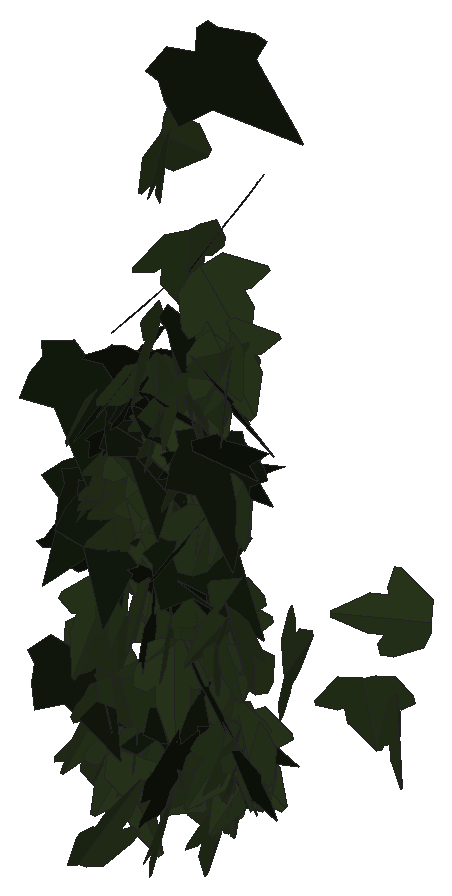
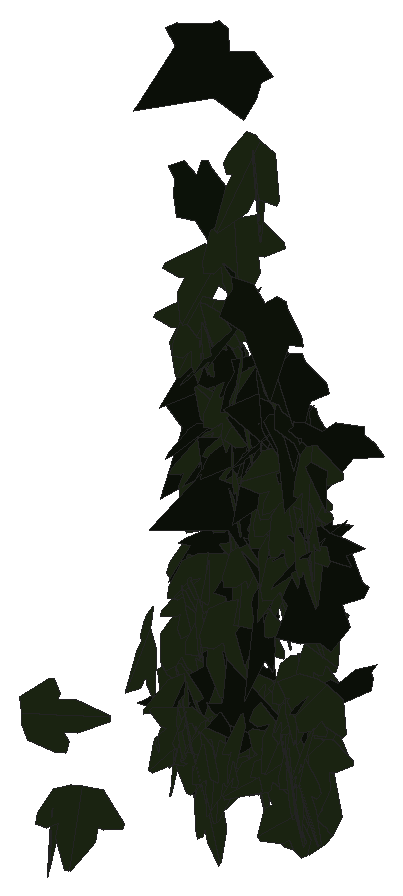
# SketchUp Ruby script. Lengths in inches.
U = 1.inch
M = Sketchup.active_model
def pt(a) = Geom::Point3d.new(a.map { |v| v * U })
def face(e, loops, mat)
  f = e.add_face(loops[0].map { |a| pt(a) })
  loops[1..].each { |l| e.add_face(l.map { |a| pt(a) }).erase! }
  f.material = f.back_material = mat if mat
  f
end
# faces: each face lists its corners as indices into pts; further lists are holes
def faces(e, pts, list, mat = nil) = list.each { |f| face(e, (f[0].is_a?(Array) ? f : [f]).map { |l| l.map { |i| pts[i] } }, mat) }
# xy, xz, yz: faces in a plane at the given z, y or x. An outline is a flat list of corners, or four numbers for a rectangle; further outlines are holes
def ring(l) = l.size == 4 ? [[l[0], l[1]], [l[2], l[1]], [l[2], l[3]], [l[0], l[3]]] : l.each_slice(2).to_a
def flat(e, list, mat, &to3) = list.each { |f| face(e, (f[0].is_a?(Array) ? f : [f]).map { |l| ring(l).map { |u, v| to3.(u, v) } }, mat) }
def xy(e, z, list, mat = nil) = flat(e, list, mat) { |x, y| [x, y, z] }
def xz(e, y, list, mat = nil) = flat(e, list, mat) { |x, z| [x, y, z] }
def yz(e, x, list, mat = nil) = flat(e, list, mat) { |y, z| [x, y, z] }
def lines(e, pts, list) = list.each { |a, b| e.add_line(pt(pts[a]), pt(pts[b])) }
# prism: a flat outline (further loops are holes) pulled along v
def prism(e, loops, v, mat = nil)
  f = face(e, loops, mat); d = Geom::Vector3d.new(v.map { |x| x * U })
  f.pushpull(f.normal.samedirection?(d) ? d.length : -d.length)
end
def box(e, o, s, mat = nil) = prism(e, [[o, [o[0] + s[0], o[1], o[2]], [o[0] + s[0], o[1] + s[1], o[2]], [o[0], o[1] + s[1], o[2]]]], [0, 0, s[2]], mat)
def at(x, y, z, deg = 0) = Geom::Transformation.translation(pt([x, y, z])) * Geom::Transformation.rotation(ORIGIN, Z_AXIS, deg.degrees)
def axes(o, x, y, z) = Geom::Transformation.new([*x, 0, *y, 0, *z, 0, *pt(o).to_a, 1])
def part(name) = M.definitions.add(name)
# library, detail: a bought-in or finely detailed component or shape, given as its bounding box
def library(name, o, s) = part(name).tap { |d| box(d.entities, o, s) }
def detail(e, o, s) = box(e.add_group.entities, o, s)
def put(e, d, t, mat = nil) = e.add_instance(d, t).tap { |i| i.material = mat if mat }
def group(e, t, mat = nil) = e.add_group.tap { |g| g.transformation = t; g.material = mat if mat }.entities
root = M.entities
M.materials.add("efeu1").color = [18, 25, 13]
M.materials.add("efeu2").color = [43, 57, 29]
c1 = part("ivyleaf_10")
p = [[0,0.5,-0.03],[-0.0625,2.02,-0.43],[-0.19,2.01,-0.46],[-0.54,1.05,-0.29],[-0.52,0.625,-0.18],[-0.83,0.76,-0.28],
  [-1.16,0.64,-0.33],[-1.15,0.33,-0.24],[-0.77,-0.39,0.02],[-0.3,-0.51,0.16],[0.04,-0.48,0.23],[-0.02,2.01,-0.4375],
  [-0.06,2.01,-0.43],[0.04,-0.49,0.23],[0.67,-0.49,0.14],[1.38,0.36,-0.2],[1.375,0.51,-0.24],[0.81,0.65,-0.19],
  [0.62,0.59,-0.15],[0.6,1.09,-0.28],[0.5,1.23,-0.31]]
faces(c1.entities,p,[[0,1,2,3,4,5,6,7,8,9,10],[11,12,0,13,14,15,16,17,18,19,20]],"efeu2")
c2 = part("ivyleaf_9")
p = [[1.54,2.16,1.25],[1.36,2.04,1.19],[-0.21,0.99,0.68],[-0.71,1.11,0.82],[-0.85,0.86,0.67],[-0.8,0.17,0.21],
  [-0.9,-0.01,0.1],[-0.67,-0.16,-0.02],[-0.08,-0.08,-0.05],[-0.03,-0.6,-0.4],[0.65,-0.88,-0.66],[0.83,-0.6,-0.49],
  [1.29,-0.42,-0.43],[1.8125,-0.07,-0.26],[1.21,0.44,0.15]]
faces(c2.entities,p,[[0,1,2,3,4,5,6,7,8,9,10,11,12,13,14]],"efeu1")
put(root,c1,axes([528.03,135.62,182.96],[0.04997,-0.69827,0.35422],[0.08449,0.35768,0.69317],[-0.77841,-0.006,0.09798]))
put(root,c1,axes([529.61,135.92,187.42],[0.72469,-0.04449,0.22869],[0.2279,-0.01976,-0.72603],[0.04837,0.75966,-0.0055]))
put(root,c1,axes([528.9,136.29,194.03],[0.25276,-0.34799,0.63465],[0.37642,-0.51097,-0.43009],[0.61821,0.4534,0.0024]))
put(root,c1,axes([529.51,135.85,184.14],[0.33931,-0.66324,-0.11644],[-0.04396,0.10828,-0.74493],[0.67195,0.342,0.01006]))
put(root,c1,axes([530.07,135.85,196.52],[-0.29708,-0.72355,-0.03236],[0.00307,0.03372,-0.7821],[0.72427,-0.29693,-0.00996]))
put(root,c2,axes([529.02,135.63,193.63],[-0.35835,0.68144,0.00431],[-0.00194,0.00385,-0.76992],[-0.68145,-0.35835,-0.00007]))
put(root,c2,axes([528.0625,136.24,189.86],[-0.09573,-0.76291,0.03566],[-0.00925,-0.03478,-0.76887],[0.76368,-0.09605,-0.00484]))
put(root,c1,axes([530.85,135.84,194.17],[-0.33415,-0.69594,-0.06383],[0.02014,0.06113,-0.77196],[0.69857,-0.33466,-0.00827]))
put(root,c1,axes([530.79,135.96,194.42],[0.72889,-0.26896,-0.11241],[-0.11049,0.02521,-0.77679],[0.26976,0.73707,-0.01445]))
put(root,c2,axes([530.46,135.66,187.6],[0.61618,-0.18002,-0.4099],[-0.39326,0.11558,-0.64194],[0.21393,0.73098,0.00055]))
put(root,c1,axes([528.93,135.89,188.72],[0.50162,-0.56592,-0.14151],[-0.06119,0.13455,-0.75503],[0.58012,0.50353,0.04271]))
put(root,c2,axes([529.75,135.23,184.89],[0.11701,0.22287,0.77167],[0.25966,0.72745,-0.24947],[-0.76008,0.28282,0.03357]))
put(root,c2,axes([528.97,136.23,192.11],[0.02537,-0.77043,-0.00224],[0.0001,0.00225,-0.77085],[0.77043,0.02537,0.00018]))
put(root,c1,axes([529.53,135.83,198.48],[0.37198,-0.66538,-0.21572],[-0.02506,0.23149,-0.75724],[0.69902,0.36238,0.08764]))
put(root,c2,axes([531.18,135.74,197.48],[-0.37583,0.69191,-0.09076],[0.04527,-0.0787,-0.78739],[-0.69637,-0.37854,-0.00221]))
put(root,c1,axes([529.17,135.92,193.36],[-0.39,-0.67294,-0.075],[0.08819,0.03533,-0.77559],[0.67133,-0.39557,0.05832]))
put(root,c1,axes([529.33,135.96,191.46],[-0.5995,-0.44929,0.13192],[-0.10238,-0.08335,-0.74915],[0.45692,-0.60816,0.00522]))
put(root,c1,axes([530.89,135.93,193.89],[0.52139,-0.58398,-0.08529],[0.04954,0.15671,-0.77016],[0.5881,0.50454,0.14049]))
put(root,c2,axes([530.53,135.64,200.75],[-0.06948,-0.12915,-0.8626],[0.43398,0.74549,-0.14658],[0.75658,-0.43948,0.00486]))
put(root,c1,axes([529.35,136.1,192.375],[0.26076,-0.72266,0.08953],[0.02445,-0.08636,-0.76825],[0.72778,0.26183,-0.00627]))
put(root,c1,axes([527.51,136.42,187.68],[-0.1066,-0.48141,0.55439],[0.28284,-0.54389,-0.41791],[0.67757,0.1513,0.26167]))
put(root,c2,axes([527.46,136.17,192.83],[-0.4125,-0.54509,-0.36487],[0.22909,0.28415,-0.68351],[0.61463,-0.47174,0.00989]))
put(root,c1,axes([529.62,135.74,193.27],[0.3847,-0.29258,-0.59439],[-0.40569,0.43936,-0.47883],[0.52376,0.55521,0.06569]))
put(root,c2,axes([530.5,136.21,192.05],[0.04603,-0.75714,-0.1445],[-0.01125,0.14409,-0.75853],[0.77073,0.04732,-0.00244]))
put(root,c1,axes([529.96,135.9,193.46],[-0.58466,0.51066,-0.08668],[0.06952,-0.05216,-0.77625],[-0.51327,-0.58874,-0.0064]))
put(root,c2,axes([527.22,136,186.73],[0.15379,-0.64621,-0.38759],[-0.0269,0.39062,-0.66193],[0.75305,0.14593,0.05551]))
put(root,c1,axes([527.78,136.29,185.7],[0.08487,0.5669,-0.472],[-0.26058,-0.42144,-0.55304],[-0.69012,0.22885,0.15077]))
put(root,c2,axes([530.27,135.87,193.9],[0.74862,-0.18729,-0.03452],[-0.03313,0.00981,-0.77169],[0.18754,0.74935,0.00147]))
put(root,c1,axes([530.96,136.07,191.26],[0.66168,-0.34231,-0.13025],[-0.10897,0.07277,-0.74484],[0.34966,0.67044,0.01435]))
put(root,c1,axes([528.38,135.85,188.53],[0.34681,-0.3359,-0.57591],[-0.42691,0.38674,-0.48265],[0.5121,0.54989,-0.01234]))
put(root,c1,axes([529.46,136.22,190.63],[-0.48763,-0.57572,0.15636],[0.0196,-0.2173,-0.73897],[0.59625,-0.46369,0.15216]))
put(root,c1,axes([529.02,136.1,191.6],[0.52098,0.5584,-0.11091],[-0.08551,-0.07188,-0.76358],[-0.56285,0.52779,0.01335]))
put(root,c2,axes([528.375,135.72,192.74],[-0.27222,0.69051,0.18515],[-0.08322,0.16617,-0.74206],[-0.71005,-0.2842,0.01599]))
put(root,c2,axes([527.84,136.42,190.25],[-0.67175,-0.3612,-0.01235],[0.01123,0.00519,-0.76271],[0.36124,-0.67185,0.00075]))
put(root,c1,axes([528.71,136.18,190.59],[-0.20937,-0.74045,0.0741],[-0.00139,-0.07659,-0.76923],[0.74414,-0.20847,0.01941]))
put(root,c1,axes([530.27,136.25,190.44],[-0.42889,-0.59636,0.21067],[-0.0606,-0.21463,-0.73091],[0.62957,-0.42692,0.07317]))
put(root,c2,axes([528.71,136.16,192.4],[0.25455,-0.68257,-0.23231],[0.01088,0.24997,-0.72254],[0.72094,0.23723,0.09293]))
put(root,c1,axes([528.48,136.29,189.77],[-0.11758,-0.7354,0.18371],[-0.00195,-0.18561,-0.74427],[0.758,-0.11455,0.02659]))
put(root,c1,axes([530.52,136.65,188.51],[0.05898,-0.24793,0.70378],[0.16298,-0.68465,-0.25484],[0.72815,0.17332,0.00004]))
put(root,c1,axes([530.69,136.4,185.81],[0.23583,0.47254,-0.49065],[-0.26364,-0.41545,-0.52682],[-0.62811,0.35179,0.03691]))
put(root,c2,axes([528.9,136.23,192.41],[0.51449,-0.57132,0.06293],[0.08496,-0.00793,-0.76667],[0.56846,0.51827,0.05764]))
put(root,c2,axes([529.85,136.1,194.64],[0.5184,-0.54014,-0.2023],[-0.09078,0.19221,-0.7458],[0.56959,0.52222,0.06526]))
put(root,c2,axes([530.13,135.85,190.32],[-0.29549,0.69132,0.10974],[-0.06843,0.09002,-0.75133],[-0.69662,-0.30208,0.02725]))
put(root,c2,axes([527.55,136.41,190.07],[0.14138,-0.74677,-0.04956],[0.02073,0.05432,-0.75943],[0.74813,0.13961,0.03041]))
put(root,c1,axes([529.43,136.16,191.8],[-0.57916,-0.4464,-0.25896],[0.33107,-0.02278,-0.70116],[0.39588,-0.63401,0.20752]))
put(root,c1,axes([529.73,136.125,192.91],[-0.36238,-0.6775,-0.10906],[0.04795,0.09803,-0.76832],[0.68455,-0.36552,-0.00392]))
put(root,c2,axes([528.93,135.93,193.67],[0.25115,0.63308,-0.36755],[-0.35506,-0.23447,-0.64646],[-0.64017,0.37841,0.21435]))
put(root,c1,axes([530.8,135.91,194.47],[0.36207,0.61508,0.32751],[0.08867,0.32541,-0.70917],[-0.69117,0.36396,0.08058]))
put(root,c2,axes([528.73,135.59,192.36],[-0.22363,0.72543,-0.3368],[-0.19552,0.28952,0.75342],[0.77553,0.28217,0.09283]))
put(root,c1,axes([529.78,135.91,191.94],[0.55958,0.2124,-0.49753],[0.43918,0.2396,0.59624],[0.31587,-0.70941,0.05241]))
put(root,c1,axes([530.59,135.9,195.76],[0.28328,0.64872,0.34617],[0.0998,0.33362,-0.70686],[-0.7285,0.29796,0.03777]))
put(root,c1,axes([528.43,136.24,190.9],[-0.27451,-0.70599,-0.01567],[0.01029,0.01282,-0.75747],[0.70609,-0.27465,0.00494]))
put(root,c1,axes([528.42,136.3,191.43],[-0.14221,-0.75335,0.02688],[-0.00755,-0.02593,-0.76665],[0.75379,-0.14238,-0.00261]))
put(root,c1,axes([529.17,136.19,192.53],[0.39766,-0.64727,-0.14511],[0.0143,0.17751,-0.75262],[0.66318,0.38429,0.10323]))
put(root,c2,axes([530.32,135.82,192.09],[0.62969,0.41873,0.08048],[0.08001,0.02495,-0.75584],[-0.41882,0.63432,-0.0234]))
put(root,c2,axes([529.03,135.92,192.73],[0.77179,0.05925,-0.00001],[-0.00778,0.10124,-0.76737],[-0.05874,0.76512,0.10154]))
put(root,c2,axes([529.51,135.97,188.96],[0.49836,0.36695,-0.44053],[-0.43808,-0.13283,-0.60623],[-0.36986,0.65176,0.12447]))
put(root,c2,axes([528.67,135.68,192.23],[0.38998,0.68815,0.26433],[0.12736,0.23165,-0.79097],[-0.72609,0.41023,0.00323]))
put(root,c1,axes([529.85,136.22,193.66],[-0.5637,0.51328,-0.09591],[0.05391,-0.08318,-0.76197],[-0.51938,-0.56572,0.02501]))
put(root,c1,axes([528.91,136.46,189.46],[-0.60638,-0.43398,0.13134],[0.03555,-0.26416,-0.70869],[0.45203,-0.56139,0.23193]))
put(root,c2,axes([529.3,135.86,195.12],[-0.05811,0.75019,0.17904],[-0.11387,0.16924,-0.74607],[-0.76281,-0.08242,0.09774]))
put(root,c1,axes([529.67,136.27,191.55],[0.26935,-0.70136,-0.16635],[0.00062,0.17781,-0.74867],[0.72081,0.26193,0.0628]))
put(root,c1,axes([528.15,136.37,190.64],[-0.07125,-0.75951,0.00136],[0.00045,-0.00141,-0.76285],[0.75951,-0.07125,0.00058]))
put(root,c1,axes([528.78,136.23,192.38],[-0.7156,-0.17808,-0.21029],[0.21261,0.01545,-0.73659],[0.1753,-0.74569,0.03496]))
put(root,c1,axes([529.57,135.88,198.61],[-0.11354,-0.54971,-0.65849],[0.11102,0.64923,-0.56112],[0.85057,-0.15813,-0.01466]))
put(root,c1,axes([527.7,136.35,190.98],[0.5122,-0.5653,-0.05899],[0.06025,0.13296,-0.75106],[0.56517,0.49815,0.13353]))
put(root,c1,axes([527.71,136.35,185.03],[-0.25185,-0.68607,-0.04226],[-0.00757,0.04777,-0.73045],[0.68732,-0.25086,-0.02353]))
put(root,c1,axes([529.42,136.09,188.07],[0.34741,-0.52139,-0.44504],[-0.1003,0.4549,-0.61123],[0.67812,0.3344,0.13759]))
put(root,c1,axes([529.84,136.4,190.58],[0.53487,-0.54169,-0.03414],[0.05809,0.10479,-0.75255],[0.53965,0.52562,0.11484]))
put(root,c1,axes([528.15,136.3,190.41],[-0.70715,-0.14617,-0.21647],[0.2202,0.00238,-0.72096],[0.14048,-0.73953,0.04046]))
put(root,c1,axes([528.26,136.29,186.12],[-0.76442,-0.05124,-0.02921],[0.02913,0.00226,-0.76613],[0.05129,-0.76497,-0.0003]))
put(root,c1,axes([527.7,136.45,190.35],[0.18373,-0.73548,-0.03494],[0.00533,0.03734,-0.75795],[0.73629,0.18325,0.01421]))
put(root,c1,axes([528,136.51,189.66],[-0.32839,-0.67339,0.09079],[-0.0079,-0.09705,-0.74836],[0.67943,-0.32659,0.03518]))
put(root,c2,axes([527.1,136.14,188.86],[0.48626,0.59301,-0.2851],[0.18549,0.21657,0.76687],[0.6313,-0.52041,-0.00573]))
put(root,c2,axes([529.79,136.34,189.75],[0.17541,-0.56337,-0.47937],[0.14807,0.50944,-0.54452],[0.72474,0.03227,0.22727]))
put(root,c1,axes([528.23,136.5625,184.76],[0.46324,0.44904,-0.34316],[-0.30982,-0.16931,-0.63979],[-0.47266,0.55107,0.08305]))
put(root,c1,axes([530.68,136.43,185.65],[0.12878,-0.69831,-0.12199],[0.06469,0.13505,-0.70476],[0.70593,0.11501,0.08683]))
put(root,c1,axes([530.81,136.34,188.5],[-0.66628,0.32126,0.02524],[-0.02364,0.00907,-0.73969],[-0.32138,-0.6667,0.0021]))
put(root,c1,axes([529.87,136.45,187.4375],[-0.55066,-0.49841,-0.0058],[0.00398,0.00425,-0.74272],[0.49842,-0.55068,-0.00048]))
put(root,c1,axes([527.57,136.375,192.14],[0.04773,-0.72337,-0.23496],[0.05319,0.23802,-0.72199],[0.75871,0.02882,0.0654]))
put(root,c2,axes([530.77,136.29,185.66],[0.52599,0.1335,-0.60109],[-0.59231,-0.10625,-0.54191],[-0.1682,0.79163,0.02864]))
put(root,c1,axes([530.63,136.8,187.3],[-0.30688,-0.6016,0.29864],[-0.02976,-0.31583,-0.66682],[0.67099,-0.28916,0.10701]))
put(root,c1,axes([527.85,136.49,187.05],[-0.13768,-0.70978,-0.15906],[0.0267,0.15684,-0.723],[0.72689,-0.1402,-0.00357]))
put(root,c1,axes([529.22,136.69,188.25],[-0.67751,0.21779,0.21168],[0.18545,-0.11315,0.70997],[0.24052,0.70073,0.04885]))
put(root,c1,axes([530.3,136.56,188.6875],[-0.42572,-0.60612,-0.08955],[0.11707,0.02657,-0.73637],[0.60141,-0.43423,0.07995]))
put(root,c1,axes([528.05,136.41,186.13],[-0.44859,-0.53531,-0.31249],[0.22213,0.22128,-0.69795],[0.57868,-0.49991,0.02568]))
put(root,c1,axes([530.68,137.05,184.99],[-0.24631,-0.41245,0.52778],[0.05126,-0.57229,-0.42331],[0.66786,-0.10818,0.22714]))
put(root,c1,axes([528.63,136.54,186.13],[-0.63713,0.36168,-0.0914],[0.07218,-0.05795,-0.73248],[-0.366,-0.64103,0.01465]))
put(root,c1,axes([530.52,136.39,191.52],[-0.11482,0.73255,0.17535],[-0.01593,0.17498,-0.74141],[-0.75308,-0.11539,-0.01105]))
put(root,c1,axes([530.6,136.19,187.91],[-0.06897,0.39523,0.63222],[-0.4718,0.4685,-0.34435],[-0.57733,-0.43008,0.20588]))
put(root,c1,axes([530.5,136.5,188.13],[0.06098,0.73613,0.11685],[-0.05063,0.12106,-0.73623],[-0.74362,0.05212,0.05971]))
put(root,c1,axes([529.32,136.73,187.97],[-0.62868,-0.35651,0.14177],[-0.0968,-0.11595,-0.72085],[0.37126,-0.63395,0.05212]))
put(root,c1,axes([530.36,136.71,186.03],[-0.58618,0.09175,-0.43939],[0.42024,-0.14177,-0.59024],[-0.15773,-0.71872,0.06034]))
put(root,c1,axes([530.06,136.65,185.05],[-0.05523,0.71756,-0.02859],[-0.05908,-0.03311,-0.71706],[-0.71569,-0.05264,0.0614]))
put(root,c2,axes([528.96,136.2,188.08],[-0.02587,0.08797,-0.81043],[-0.68239,0.44124,0.06968],[0.44596,0.68027,0.05961]))
put(root,c1,axes([530.92,136.78,185.92],[-0.60851,0.24593,0.34474],[-0.407,-0.17298,-0.59501],[-0.11695,-0.67765,0.277]))
put(root,c1,axes([527.17,136.79,186.86],[-0.55388,-0.24517,-0.41694],[0.46712,-0.10668,-0.55781],[0.12549,-0.68501,0.23609]))
put(root,c2,axes([529.33,136.53,186.02],[0.21467,0.06139,-0.8254],[0.56729,0.61001,0.19291],[0.60269,-0.59604,0.11241]))
put(root,c1,axes([527.67,136.83,184.71],[0.23052,-0.68202,-0.07062],[-0.00295,0.07352,-0.71963],[0.68566,0.22961,0.02064]))
put(root,c1,axes([527.77,136.86,183.7],[0.44424,-0.04921,0.57248],[0.57419,0.01099,-0.44462],[0.02146,0.72454,0.04562]))
put(root,c1,axes([530.51,136.875,185.27],[0.33571,-0.63345,-0.05716],[-0.00812,0.06036,-0.71661],[0.63598,0.33515,0.02102]))
put(root,c1,axes([530.77,136.78,185.89],[0.1058,0.7143,-0.0417],[-0.01466,-0.03998,-0.72205],[-0.71537,0.10646,0.00863]))
put(root,c2,axes([528.18,136.26,192.26],[-0.07592,0.52294,0.5575],[-0.07785,0.55204,-0.52842],[-0.7604,-0.10873,-0.00156]))
put(root,c1,axes([527.44,136.76,185.65],[-0.36548,0.631,-0.02428],[-0.00997,-0.03381,-0.72875],[-0.63139,-0.36472,0.02556]))
put(root,c2,axes([528.8,136.58,185.3],[-0.7139,0.19389,0.41929],[0.40609,-0.10451,0.73974],[0.22021,0.8213,-0.00485]))
put(root,c1,axes([527.65,136.72,184.74],[0.49961,-0.36196,-0.42016],[-0.29103,0.31027,-0.61334],[0.47207,0.57435,0.06655]))
put(root,c1,axes([529.93,137.18,184.66],[0.25178,0.2857,-0.60647],[-0.44586,-0.41243,-0.37939],[-0.50064,0.51099,0.03288]))
put(root,c1,axes([528.28,136.4,184.71],[0.22685,0.20136,0.66661],[0.278,0.61661,-0.28086],[-0.63846,0.34003,0.11456]))
put(root,c1,axes([528.34,136.3,191.76],[0.10893,-0.22987,0.78589],[-0.21987,0.75549,0.25145],[-0.78875,-0.24235,0.03844]))
put(root,c1,axes([530.44,137.07,185.33],[0.22953,-0.67108,0.12069],[0.06425,-0.10549,-0.70876],[0.67881,0.2369,0.02628]))
put(root,c1,axes([529.68,136.86,184.6],[-0.17137,-0.68086,-0.13484],[0.05378,0.12544,-0.70178],[0.69199,-0.17836,0.02115]))
put(root,c2,axes([529.43,136.26,190.89],[0.43732,0.3907,0.59865],[0.3997,0.44819,-0.5845],[-0.59268,0.59055,0.04754]))
put(root,c1,axes([529.26,136.67,185.33],[-0.29356,0.63899,0.22033],[-0.15454,0.1704,-0.70009],[-0.65801,-0.3251,0.06612]))
put(root,c1,axes([529.93,136.89,184.97],[-0.41525,-0.599,-0.06841],[0.02632,0.06498,-0.72869],[0.60232,-0.4158,-0.01532]))
put(root,c1,axes([527.99,136.75,185.3],[0.47671,-0.38712,-0.39338],[-0.1904,0.37255,-0.59734],[0.51803,0.49317,0.14246]))
put(root,c1,axes([530.07,137.11,184.87],[0.62321,-0.34286,0.12479],[0.17988,0.07383,-0.69549],[0.31744,0.63128,0.14912]))
put(root,c1,axes([527.55,137.11,185.11],[0.34384,-0.61946,-0.14752],[-0.04906,0.14138,-0.70804],[0.63489,0.34641,0.02518]))
put(root,c1,axes([530.14,137.15,184.6],[0.37262,-0.59763,-0.12575],[-0.07011,0.10447,-0.70427],[0.60668,0.37914,-0.00415]))
put(root,c1,axes([529.73,137.23,183.63],[0.11063,-0.69926,0.00613],[0.00093,-0.00606,-0.70796],[0.69929,0.11064,-0.00003]))
put(root,c1,axes([529.77,137.03,184.6],[-0.69577,0.14245,0.06295],[-0.05988,0.02136,-0.71015],[-0.14376,-0.69828,-0.00888]))
put(root,c1,axes([530.17,137.07,185.14],[0.37474,0.36428,0.49339],[0.33183,0.36583,-0.52213],[-0.51578,0.50003,0.02255]))
put(root,c1,axes([530.54,137.04,185.04],[-0.35359,0.50507,0.35484],[-0.23694,0.26655,-0.6155],[-0.56997,-0.42413,0.03573]))
put(root,c1,axes([531.125,137.48,187.12],[0.02944,-0.1645,-0.83713],[-0.14681,0.82416,-0.16711],[0.84041,0.14973,0.00013]))
put(root,c1,axes([531.36,140.89,186.71],[0.01385,0.07794,0.72358],[-0.51786,-0.50742,0.06457],[0.51133,-0.51602,0.0458]))
put(root,c1,axes([530.36,140.81,184.9],[-0.59921,-0.39726,-0.06521],[0.05507,0.03494,-0.71894],[0.39879,-0.60174,0.0013]))
put(root,c1,axes([530.76,141.15,184.4],[0.28667,-0.61256,0.19596],[0.30209,-0.06115,-0.63309],[0.56777,0.34182,0.2379]))
